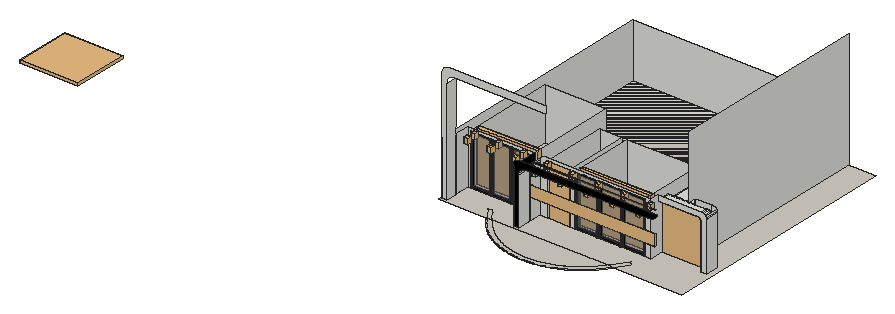
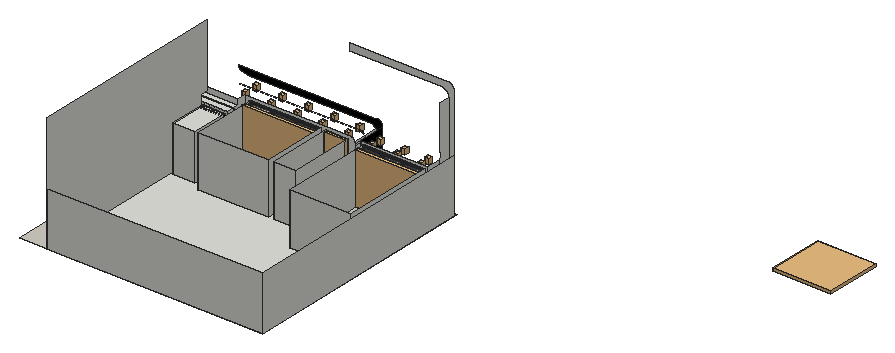
# SketchUp Ruby script. Lengths in inches.
U = 1.inch
M = Sketchup.active_model
def pt(a) = Geom::Point3d.new(a.map { |v| v * U })
def face(e, loops, mat)
  f = e.add_face(loops[0].map { |a| pt(a) })
  loops[1..].each { |l| e.add_face(l.map { |a| pt(a) }).erase! }
  f.material = f.back_material = mat if mat
  f
end
# faces: each face lists its corners as indices into pts; further lists are holes
def faces(e, pts, list, mat = nil) = list.each { |f| face(e, (f[0].is_a?(Array) ? f : [f]).map { |l| l.map { |i| pts[i] } }, mat) }
# xy, xz, yz: faces in a plane at the given z, y or x. An outline is a flat list of corners, or four numbers for a rectangle; further outlines are holes
def ring(l) = l.size == 4 ? [[l[0], l[1]], [l[2], l[1]], [l[2], l[3]], [l[0], l[3]]] : l.each_slice(2).to_a
def flat(e, list, mat, &to3) = list.each { |f| face(e, (f[0].is_a?(Array) ? f : [f]).map { |l| ring(l).map { |u, v| to3.(u, v) } }, mat) }
def xy(e, z, list, mat = nil) = flat(e, list, mat) { |x, y| [x, y, z] }
def xz(e, y, list, mat = nil) = flat(e, list, mat) { |x, z| [x, y, z] }
def yz(e, x, list, mat = nil) = flat(e, list, mat) { |y, z| [x, y, z] }
def lines(e, pts, list) = list.each { |a, b| e.add_line(pt(pts[a]), pt(pts[b])) }
# prism: a flat outline (further loops are holes) pulled along v
def prism(e, loops, v, mat = nil)
  f = face(e, loops, mat); d = Geom::Vector3d.new(v.map { |x| x * U })
  f.pushpull(f.normal.samedirection?(d) ? d.length : -d.length)
end
def box(e, o, s, mat = nil) = prism(e, [[o, [o[0] + s[0], o[1], o[2]], [o[0] + s[0], o[1] + s[1], o[2]], [o[0], o[1] + s[1], o[2]]]], [0, 0, s[2]], mat)
def at(x, y, z, deg = 0) = Geom::Transformation.translation(pt([x, y, z])) * Geom::Transformation.rotation(ORIGIN, Z_AXIS, deg.degrees)
def axes(o, x, y, z) = Geom::Transformation.new([*x, 0, *y, 0, *z, 0, *pt(o).to_a, 1])
def part(name) = M.definitions.add(name)
# library, detail: a bought-in or finely detailed component or shape, given as its bounding box
def library(name, o, s) = part(name).tap { |d| box(d.entities, o, s) }
def detail(e, o, s) = box(e.add_group.entities, o, s)
def put(e, d, t, mat = nil) = e.add_instance(d, t).tap { |i| i.material = mat if mat }
def group(e, t, mat = nil) = e.add_group.tap { |g| g.transformation = t; g.material = mat if mat }.entities
root = M.entities
M.materials.add("Arta-Ceramic-Moonstone-White-24x24-4K").color = [209, 205, 196]
M.materials.add("Glass_Tinted_Gray").color = [0, 0, 0]
M.materials["Glass_Tinted_Gray"].alpha = 0.125
M.materials.add("[0130_Gainsboro]").color = [39, 45, 50]
M.materials.add("[0135_DarkGray]").color = [81, 81, 81]
M.materials.add("[Color M00]").color = [255, 255, 255]
M.materials.add("[Color M09]").color = [0, 0, 0]
M.materials.add("[Mirror 02]").color = [229, 229, 229]
M.materials.add("[Terrazzo Light Blue]").color = [196, 214, 227]
M.materials.add("[Translucent Glass Gray]1").color = [128, 128, 128]
M.materials["[Translucent Glass Gray]1"].alpha = 0.5
c1 = library("CURTAIN",[20.4,9.88,0],[29.77,2.88,102.36])
c2 = library("door by lz",[5.91,-4.92,0],[35.43,6.61,78.74])
c3 = library("Mesh Light\#2",[-0.5,-0.5,-0.1],[1,1,0.2])
c4 = library("Group\#4",[-0.5,-0.5,0],[98.5,2,108])
c5 = part("Glazed door panel")
xy(c5.entities,0,[[0,-0.98,43.07,0],[0,0,43.07,1.4]],"[0130_Gainsboro]")
xy(c5.entities,0.3,[[0.3,-1.43,42.77,-0.98]],"[0130_Gainsboro]")
xy(c5.entities,2.95,[[2.95,-0.63,40.12,0],[2.95,0,40.12,0.64],[2.95,0.64,40.12,1.4]],"[0130_Gainsboro]")
xy(c5.entities,2.95,[[2.95,-1.43,40.12,-0.63]],"[Color M09]")
xy(c5.entities,3.54,[[3.54,0,39.53,0.64]],"[0130_Gainsboro]")
xy(c5.entities,3.54,[[3.54,-0.63,39.53,0]],"[Color M09]")
xy(c5.entities,111.8125,[[3.54,0,39.53,0.64]],"[0130_Gainsboro]")
xy(c5.entities,111.8125,[[3.54,-0.63,39.53,0]],"[Color M09]")
xy(c5.entities,112.4,[[2.95,-0.63,40.12,0],[2.95,0,40.12,0.64],[2.95,0.64,40.12,1.4]],"[0130_Gainsboro]")
xy(c5.entities,112.4,[[2.95,-1.43,40.12,-0.63]],"[Color M09]")
xy(c5.entities,115.05,[[0.3,-1.43,42.77,-0.98]],"[0130_Gainsboro]")
xy(c5.entities,115.35,[[0,-0.98,43.07,0],[0,0,43.07,1.4]],"[0130_Gainsboro]")
xz(c5.entities,-1.43,[[[0.3,0.3,42.77,115.05],[2.95,2.95,40.12,112.4]]],"[Color M09]")
xz(c5.entities,-0.98,[[[0,0,43.07,115.35],[0.3,0.3,42.77,115.05]]],"[Color M00]")
xz(c5.entities,-0.63,[[[2.95,2.95,40.12,112.4],[3.54,3.54,39.53,111.8125]]],"[Color M09]")
xz(c5.entities,0,[[[0,0,43.07,115.35],[2.95,2.95,40.12,112.4]],[[2.95,2.95,40.12,112.4],[3.54,3.54,39.53,111.8125]]],"[0130_Gainsboro]")
xz(c5.entities,0,[[3.54,3.54,39.53,111.8125]],"[Translucent Glass Gray]1")
xz(c5.entities,0.64,[[[2.95,2.95,40.12,112.4],[3.54,3.54,39.53,111.8125]]],"[0130_Gainsboro]")
xz(c5.entities,1.4,[[[0,0,43.07,115.35],[2.95,2.95,40.12,112.4]]],"[0130_Gainsboro]")
yz(c5.entities,0,[[-0.98,0,0,115.35],[0,0,1.4,115.35]],"[0130_Gainsboro]")
yz(c5.entities,0.3,[[-1.43,0.3,-0.98,115.05]],"[Color M00]")
yz(c5.entities,2.95,[[-0.63,2.95,0,112.4],[0,2.95,0.64,112.4],[0.64,2.95,1.4,112.4]],"[0130_Gainsboro]")
yz(c5.entities,2.95,[[-1.43,2.95,-0.63,112.4]],"[Color M09]")
yz(c5.entities,3.54,[[0,3.54,0.64,111.8125]],"[0130_Gainsboro]")
yz(c5.entities,3.54,[[-0.63,3.54,0,111.8125]],"[Color M09]")
yz(c5.entities,39.53,[[0,3.54,0.64,111.8125]],"[0130_Gainsboro]")
yz(c5.entities,39.53,[[-0.63,3.54,0,111.8125]],"[Color M09]")
yz(c5.entities,40.12,[[-0.63,2.95,0,112.4],[0,2.95,0.64,112.4],[0.64,2.95,1.4,112.4]],"[0130_Gainsboro]")
yz(c5.entities,40.12,[[-1.43,2.95,-0.63,112.4]],"[Color M09]")
yz(c5.entities,42.77,[[-1.43,0.3,-0.98,115.05]],"[Color M00]")
yz(c5.entities,43.07,[[-0.98,0,0,115.35],[0,0,1.4,115.35]],"[0130_Gainsboro]")
c6 = part("Sliding glass doors")
put(c6.entities,c5,axes([90.57,1.43,0],[1.05148,0,0],[0,1,0],[0,0,1]),"[Color M09]")
put(c6.entities,c5,axes([0,1.43,0],[1.05148,0,0],[0,1,0],[0,0,1]))
put(c6.entities,c5,axes([45.29,1.43,0],[1.05148,0,0],[0,1,0],[0,0,1]))
c7 = part("PENTEK_RP Fineline 50S_Sliding_DoorCase_E1")
xy(c7.entities,0,[[0,0,1.51,3.66]],"[Color M09]")
xy(c7.entities,99.27,[[0,0,1.51,3.66]],"[Color M09]")
xz(c7.entities,0,[[0,0,1.51,99.27]],"[Color M09]")
xz(c7.entities,3.66,[[0,0,1.51,99.27]],"[0135_DarkGray]")
yz(c7.entities,0,[[0,0,3.66,99.27]],"[Color M09]")
yz(c7.entities,1.51,[[0,0,3.66,99.27]],"[Color M09]")
c8 = part("PENTEK_RP Fineline 50S_SlidingDooe_Case_E2")
xy(c8.entities,0,[[0,0,96.25,3.66]],"[Color M09]")
xy(c8.entities,1.51,[[0,0,96.25,3.66]],"[Color M09]")
xz(c8.entities,0,[[0,0,96.25,1.51]],"[Color M09]")
xz(c8.entities,3.66,[[0,0,96.25,1.51]],"[0135_DarkGray]")
yz(c8.entities,0,[[0,0,3.66,1.51]],"[Color M09]")
yz(c8.entities,96.25,[[0,0,3.66,1.51]],"[Color M09]")
c9 = part("pentek_RP Fineline 50S_SlidingDoor_Case")
put(c9.entities,c7,at(97.76,0,0))
put(c9.entities,c8,at(1.51,0,0))
put(c9.entities,c7,at(0,0,0))
put(c9.entities,c8,at(1.51,0,97.76))
c10 = part("PENTEK_RP Fineline 50S_SlidingDoor_GlazingBead_2")
xy(c10.entities,0,[[0,0,0.56,0.59]],"[0135_DarkGray]")
xy(c10.entities,94.39,[[0,0,0.56,0.59]],"[0135_DarkGray]")
xz(c10.entities,0,[[0,0,0.56,94.39]],"[Color M09]")
xz(c10.entities,0.59,[[0,0,0.56,94.39]],"[0135_DarkGray]")
yz(c10.entities,0,[[0,0,0.59,94.39]],"[0135_DarkGray]")
yz(c10.entities,0.56,[[0,0,0.59,94.39]],"[Color M09]")
c11 = part("PENTEK_RP Fineline 50S_SlidingDoor_Glass")
box(c11.entities,[0,0,0],[46.58,0.16,94.39],"Glass_Tinted_Gray")
c12 = part("PENTEK_RP Fineline 50S_SlidingDoor_GlazingBead")
box(c12.entities,[0,0,0],[45.47,0.59,0.56],"[Color M09]")
c13 = part("PENTEK_RP Fineline 50S_SlidingDoor_Leaf_E1")
xy(c13.entities,0,[[0,0,0.93,1.97],[0.93,1.57,1.49,1.97]],"[0135_DarkGray]")
xy(c13.entities,96.25,[[0,0,0.93,0,0.93,1.57,1.49,1.57,1.49,1.97,0,1.97]],"[0135_DarkGray]")
xz(c13.entities,0,[[0,0,0.93,96.25]],"[Color M09]")
xz(c13.entities,1.57,[[0.93,0,1.49,95.32],[0.93,95.32,1.49,96.25]],"[0135_DarkGray]")
xz(c13.entities,1.97,[[0,0,1.49,96.25]],"[0135_DarkGray]")
yz(c13.entities,0,[[0,0,1.97,96.25]],"[Color M09]")
yz(c13.entities,0.93,[[0,0,1.57,0.93],[0,95.32,1.57,96.25]],"[0135_DarkGray]")
yz(c13.entities,0.93,[[0,0.93,1.57,95.32]],"[Color M09]")
yz(c13.entities,1.49,[[1.57,0,1.97,95.32],[1.57,95.32,1.97,96.25]],"[0135_DarkGray]")
c14 = part("PENTEK_RP Fineline 50S_SlidingDoor_Leaf_E2")
xy(c14.entities,0,[[0,0,0,1.57,0.56,1.57,0.56,1.97,46.02,1.97,46.02,1.57,46.58,1.57,46.58,0]],"[Color M09]")
xy(c14.entities,0.93,[[0,0,46.58,1.57]],"[Color M09]")
xy(c14.entities,1.49,[[0.56,1.57,46.02,1.97]],"[Color M09]")
xz(c14.entities,0,[[0,0,46.58,0.93]],"[Color M09]")
xz(c14.entities,1.57,[[0,0,0.56,0.93],[46.02,0,46.58,0.93]],"[0135_DarkGray]")
xz(c14.entities,1.57,[[0.56,0.93,46.02,1.49]],"[Color M09]")
xz(c14.entities,1.97,[[0.56,0,46.02,1.49]],"[0135_DarkGray]")
yz(c14.entities,0,[[0,0,1.57,0.93]],"[Color M09]")
yz(c14.entities,0.56,[[1.57,0,1.97,0.93]],"[0135_DarkGray]")
yz(c14.entities,0.56,[[1.57,0.93,1.97,1.49]],"[Color M09]")
yz(c14.entities,46.02,[[1.57,0,1.97,0.93]],"[0135_DarkGray]")
yz(c14.entities,46.02,[[1.57,0.93,1.97,1.49]],"[Color M09]")
yz(c14.entities,46.58,[[0,0,1.57,0.93]],"[Color M09]")
c15 = part("PENTEK_RP Fineline S_SlidingDoor_Leaf1")
put(c15.entities,c10,at(0.93,0,0.93))
put(c15.entities,c10,at(46.96,0,0.93))
put(c15.entities,c11,at(1.49,1.42,0.93))
put(c15.entities,c12,at(1.49,0,0.93))
put(c15.entities,c11,at(1.49,0.59,0.93),"[Terrazzo Light Blue]")
put(c15.entities,c13,at(0,0,0))
put(c15.entities,c13,axes([48.44,0,0],[-1,0,0],[0,1,0],[0,0,1]))
put(c15.entities,c14,axes([0.93,0,96.25],[1,0,0],[0,1,0],[0,0,-1]))
put(c15.entities,c14,at(0.93,0,0))
put(c15.entities,c12,at(1.49,0,94.77))
c16 = part("PENTEK_RP Fineline 50S_SlidingDoor_Leaf2")
put(c16.entities,c11,at(1.49,1.42,0.93))
put(c16.entities,c12,at(1.49,0,94.77))
put(c16.entities,c10,at(46.96,0,0.93))
put(c16.entities,c11,at(1.49,0.59,0.93),"[Mirror 02]")
put(c16.entities,c10,at(0.93,0,0.93))
put(c16.entities,c13,at(0,0,0))
put(c16.entities,c13,axes([48.44,0,0],[-1,0,0],[0,1,0],[0,0,1]))
put(c16.entities,c12,at(1.49,0,0.93))
put(c16.entities,c14,axes([0.93,0,96.25],[1,0,0],[0,1,0],[0,0,-1]))
put(c16.entities,c14,at(0.93,0,0))
c17 = part("PENTEK - Slimmest Steel Sliding Door / Window\#2")
put(c17.entities,c9,at(0,-1.88,-0.09),"[Color M09]")
put(c17.entities,c15,at(1.51,-2.27,1.42))
put(c17.entities,c16,at(49.32,-0.3,1.42))
c18 = library("Curtains",[0,0,0],[121.73,8.19,117.22])
c19 = library("Group\#166",[0,0,0],[129,124.5,6])
c20 = library("IES Light",[-4.45,-4.45,-12],[8.9,8.9,12])
xy(root,30,[[777.4375,202.125,777.4375,734.875,1257.4375,734.875,1257.4375,307.9375,1251.4375,307.9375,1251.4375,391.375,1202.71,391.375,1202.71,307.9375,1196.71,307.9375,1196.71,260.875,1183.9375,260.875,1183.9375,406.0625,1027.75,406.0625,1027.75,260.875,1015.75,260.875,1015.75,406.0625,967.75,406.0625,967.75,260.875,949.4375,260.875,949.4375,202.125,937.4375,202.125,937.4375,260.875,931.4375,260.875,931.4375,467.3125,795.4375,467.3125,795.4375,260.875,789.4375,260.875,789.4375,202.125],[1294.21,278.875,1306.21,307.9375]])
xy(root,30,[[1024.28,117.49,1027.49,117.52,1030.7,117.61,1033.91,117.77,1037.12,117.98,1040.32,118.26,1043.51,118.6,1046.7,119,1049.88,119.46,1053.05,119.98,1056.21,120.5625,1059.36,121.2,1062.49,121.91,1065.61,122.67,1068.72,123.49,1071.81,124.375,1074.875,125.32,1077.93,126.32,1080.96,127.375,1083.97,128.49,1086.97,129.67,1089.93,130.9,1092.875,132.1875,1095.79,133.53,1098.68,134.93,1101.55,136.38,1104.38,137.89,1107.19,139.46,1109.97,141.08,1112.71,142.75,1115.42,144.47,1118.1,146.24,1120.74,148.07,1123.35,149.94,1125.92,151.87,1128.46,153.84,1130.95,155.87,1133.41,157.9375,1135.82,160.05,1138.2,162.22,1140.53,164.43,1142.82,166.68,1145.07,168.97,1147.27,171.3125,1149.43,173.69,1151.54,176.12,1153.6,178.58,1155.62,181.08,1157.59,183.62,1159.51,186.19,1165.71,194.86,1165.69,194.875,1164.72,194.875,1158.85,186.67,1156.94,184.11,1154.98,181.58,1152.97,179.09,1150.92,176.64,1148.82,174.23,1146.67,171.87,1144.48,169.54,1142.25,167.25,1139.97,165.01,1137.64,162.8125,1135.28,160.66,1132.875,158.55,1130.43,156.49,1127.95,154.48,1125.43,152.52,1122.87,150.6,1120.27,148.73,1117.64,146.92,1114.98,145.15,1112.28,143.4375,1109.55,141.77,1106.79,140.16,1103.99,138.61,1101.17,137.11,1098.32,135.66,1095.45,134.27,1092.54,132.93,1089.61,131.65,1086.66,130.42,1083.68,129.25,1080.6875,128.14,1077.67,127.09,1074.63,126.09,1071.57,125.16,1068.5,124.28,1065.41,123.46,1062.31,122.7,1059.1875,122,1056.05,121.36,1052.91,120.78,1049.76,120.26,1046.59,119.8,1043.42,119.41,1040.24,119.07,1037.06,118.79,1033.87,118.58,1030.67,118.43,1027.48,118.33,1024.28,118.3,1021.08,118.33,1017.89,118.43,1014.7,118.58,1011.51,118.79,1008.32,119.07,1005.14,119.41,1001.97,119.8,998.81,120.26,995.65,120.78,992.51,121.36,989.375,122,986.26,122.7,983.15,123.46,980.0625,124.28,976.99,125.16,973.93,126.09,970.89,127.09,967.875,128.14,964.875,129.25,961.9,130.42,958.95,131.65,956.02,132.93,953.12,134.27,950.24,135.66,947.39,137.11,944.57,138.61,941.77,140.16,939.01,141.77,936.28,143.4375,933.58,145.15,930.92,146.92,928.29,148.73,925.69,150.6,923.13,152.52,920.61,154.48,918.13,156.49,915.68,158.55,913.28,160.66,910.92,162.8125,908.59,165.01,906.32,167.25,904.08,169.54,901.89,171.87,899.74,174.23,897.64,176.64,895.59,179.09,893.58,181.58,891.62,184.11,889.71,186.67,883.84,194.875,882.84,194.875,889.06,186.19,890.97,183.62,892.94,181.08,894.96,178.58,897.02,176.12,899.13,173.69,901.29,171.3125,903.49,168.97,905.74,166.68,908.03,164.43,910.36,162.22,912.74,160.05,915.15,157.9375,917.61,155.87,920.11,153.84,922.64,151.87,925.21,149.94,927.82,148.07,930.46,146.24,933.14,144.47,935.85,142.75,938.6,141.08,941.37,139.46,944.18,137.89,947.01,136.38,949.88,134.93,952.77,133.53,955.6875,132.1875,958.63,130.9,961.6,129.67,964.59,128.49,967.6,127.375,970.63,126.32,973.68,125.32,976.76,124.375,979.85,123.49,982.95,122.67,986.07,121.91,989.21,121.2,992.35,120.5625,995.51,119.98,998.68,119.46,1001.86,119,1005.05,118.6,1008.24,118.26,1011.44,117.98,1014.65,117.77,1017.86,117.61,1021.07,117.52],[1024.28,118.3,1027.48,118.33,1030.67,118.43,1033.87,118.58,1037.06,118.79,1040.24,119.07,1043.42,119.41,1046.59,119.8,1049.76,120.26,1052.91,120.78,1056.05,121.36,1059.1875,122,1062.31,122.7,1065.41,123.46,1068.5,124.28,1071.57,125.16,1074.63,126.09,1077.67,127.09,1080.6875,128.14,1083.68,129.25,1086.66,130.42,1089.61,131.65,1092.54,132.93,1095.45,134.27,1098.32,135.66,1101.17,137.11,1103.99,138.61,1106.79,140.16,1109.55,141.77,1112.28,143.4375,1114.98,145.15,1117.64,146.92,1120.27,148.73,1122.87,150.6,1125.43,152.52,1127.95,154.48,1130.43,156.49,1132.875,158.55,1135.28,160.66,1137.64,162.8125,1139.97,165.01,1142.25,167.25,1144.48,169.54,1146.67,171.87,1148.82,174.23,1150.92,176.64,1152.97,179.09,1154.98,181.58,1156.94,184.11,1158.85,186.67,1164.72,194.875,1152.72,194.875,1150.98,192.41,1149.2,189.97,1147.37,187.57,1145.49,185.21,1143.57,182.88,1141.61,180.59,1139.59,178.34,1137.54,176.125,1135.45,173.95,1133.31,171.82,1131.13,169.73,1128.91,167.6875,1126.65,165.68,1124.36,163.72,1122.02,161.81,1119.65,159.94,1117.25,158.12,1114.81,156.34,1112.33,154.61,1109.83,152.93,1107.29,151.3,1104.72,149.72,1102.12,148.19,1099.49,146.71,1096.83,145.28,1094.14,143.9,1091.43,142.57,1088.69,141.3,1085.93,140.08,1083.15,138.91,1080.34,137.8,1077.52,136.74,1074.67,135.74,1071.81,134.79,1068.92,133.9,1066.02,133.07,1063.11,132.29,1060.18,131.5625,1057.23,130.9,1054.28,130.29,1051.31,129.74,1048.33,129.24,1045.34,128.81,1042.35,128.43,1039.35,128.11,1036.34,127.84,1033.33,127.64,1030.32,127.49,1027.3,127.41,1024.28,127.375,1021.26,127.41,1018.25,127.49,1015.23,127.64,1012.22,127.84,1009.21,128.11,1006.21,128.43,1003.22,128.81,1000.23,129.24,997.25,129.74,994.29,130.29,991.33,130.9,988.39,131.5625,985.46,132.29,982.54,133.07,979.64,133.9,976.76,134.79,973.89,135.74,971.04,136.74,968.22,137.8,965.41,138.91,962.63,140.08,959.87,141.3,957.13,142.57,954.42,143.9,951.73,145.28,949.08,146.71,946.45,148.19,943.85,149.72,941.27,151.3,938.74,152.93,936.23,154.61,933.75,156.34,931.3125,158.12,928.91,159.94,926.54,161.81,924.2,163.72,921.91,165.68,919.65,167.6875,917.43,169.73,915.25,171.82,913.12,173.95,911.02,176.125,908.97,178.34,906.96,180.59,904.99,182.88,903.07,185.21,901.19,187.57,899.36,189.97,897.58,192.41,895.84,194.875,883.84,194.875,889.71,186.67,891.62,184.11,893.58,181.58,895.59,179.09,897.64,176.64,899.74,174.23,901.89,171.87,904.08,169.54,906.32,167.25,908.59,165.01,910.92,162.8125,913.28,160.66,915.68,158.55,918.13,156.49,920.61,154.48,923.13,152.52,925.69,150.6,928.29,148.73,930.92,146.92,933.58,145.15,936.28,143.4375,939.01,141.77,941.77,140.16,944.57,138.61,947.39,137.11,950.24,135.66,953.12,134.27,956.02,132.93,958.95,131.65,961.9,130.42,964.875,129.25,967.875,128.14,970.89,127.09,973.93,126.09,976.99,125.16,980.0625,124.28,983.15,123.46,986.26,122.7,989.375,122,992.51,121.36,995.65,120.78,998.81,120.26,1001.97,119.8,1005.14,119.41,1008.32,119.07,1011.51,118.79,1014.7,118.58,1017.89,118.43,1021.08,118.33],[1024.28,127.375,1027.3,127.41,1030.32,127.49,1033.33,127.64,1036.34,127.84,1039.35,128.11,1042.35,128.43,1045.34,128.81,1048.33,129.24,1051.31,129.74,1054.28,130.29,1057.23,130.9,1060.18,131.5625,1063.11,132.29,1066.02,133.07,1068.92,133.9,1071.81,134.79,1074.67,135.74,1077.52,136.74,1080.34,137.8,1083.15,138.91,1085.93,140.08,1088.69,141.3,1091.43,142.57,1094.14,143.9,1096.83,145.28,1099.49,146.71,1102.12,148.19,1104.72,149.72,1107.29,151.3,1109.83,152.93,1112.33,154.61,1114.81,156.34,1117.25,158.12,1119.65,159.94,1122.02,161.81,1124.36,163.72,1126.65,165.68,1128.91,167.6875,1131.13,169.73,1133.31,171.82,1135.45,173.95,1137.54,176.125,1139.59,178.34,1141.61,180.59,1143.57,182.88,1145.49,185.21,1147.37,187.57,1149.2,189.97,1150.98,192.41,1152.72,194.875,1150.97,192.43,1149.17,190.01,1147.33,187.64,1145.4375,185.29,1143.5,182.99,1141.52,180.72,1139.5,178.49,1137.44,176.3,1135.34,174.15,1133.19,172.04,1131,169.97,1128.78,167.94,1126.52,165.96,1124.21,164.02,1121.875,162.12,1119.5,160.27,1117.09,158.47,1114.65,156.71,1112.17,155,1109.67,153.34,1107.125,151.72,1104.55,150.16,1101.95,148.64,1099.33,147.18,1096.67,145.76,1093.99,144.4,1091.28,143.09,1088.54,141.83,1085.79,140.625,1083.01,139.47,1080.21,138.37,1077.38,137.32,1074.54,136.33,1071.68,135.4,1068.8,134.51,1065.91,133.6875,1063,132.92,1060.08,132.2,1057.14,131.54,1054.19,130.94,1051.23,130.4,1048.26,129.91,1045.28,129.48,1042.3,129.1,1039.31,128.78,1036.31,128.52,1033.3,128.32,1030.3,128.18,1027.29,128.09,1024.28,128.0625,1021.27,128.09,1018.26,128.18,1015.26,128.32,1012.25,128.52,1009.26,128.78,1006.26,129.1,1003.28,129.48,1000.3,129.91,997.33,130.4,994.37,130.94,991.42,131.54,988.48,132.2,985.56,132.92,982.65,133.6875,979.76,134.51,976.88,135.4,974.02,136.33,971.18,137.32,968.36,138.37,965.56,139.47,962.78,140.625,960.02,141.83,957.28,143.09,954.58,144.4,951.89,145.76,949.24,147.18,946.61,148.64,944.01,150.16,941.4375,151.72,938.9,153.34,936.39,155,933.91,156.71,931.47,158.47,929.06,160.27,926.69,162.12,924.35,164.02,922.05,165.96,919.78,167.94,917.56,169.97,915.37,172.04,913.23,174.15,911.12,176.3,909.06,178.49,907.04,180.72,905.06,182.99,903.125,185.29,901.24,187.64,899.39,190.01,897.59,192.43,895.84,194.875,897.58,192.41,899.36,189.97,901.19,187.57,903.07,185.21,904.99,182.88,906.96,180.59,908.97,178.34,911.02,176.125,913.12,173.95,915.25,171.82,917.43,169.73,919.65,167.6875,921.91,165.68,924.2,163.72,926.54,161.81,928.91,159.94,931.3125,158.12,933.75,156.34,936.23,154.61,938.74,152.93,941.27,151.3,943.85,149.72,946.45,148.19,949.08,146.71,951.73,145.28,954.42,143.9,957.13,142.57,959.87,141.3,962.63,140.08,965.41,138.91,968.22,137.8,971.04,136.74,973.89,135.74,976.76,134.79,979.64,133.9,982.54,133.07,985.46,132.29,988.39,131.5625,991.33,130.9,994.29,130.29,997.25,129.74,1000.23,129.24,1003.22,128.81,1006.21,128.43,1009.21,128.11,1012.22,127.84,1015.23,127.64,1018.25,127.49,1021.26,127.41],[1024.28,128.0625,1027.29,128.09,1030.3,128.18,1033.3,128.32,1036.31,128.52,1039.31,128.78,1042.3,129.1,1045.28,129.48,1048.26,129.91,1051.23,130.4,1054.19,130.94,1057.14,131.54,1060.08,132.2,1063,132.92,1065.91,133.6875,1068.8,134.51,1071.68,135.4,1074.54,136.33,1077.38,137.32,1080.21,138.37,1083.01,139.47,1085.79,140.625,1088.54,141.83,1091.28,143.09,1093.99,144.4,1096.67,145.76,1099.33,147.18,1101.95,148.64,1104.55,150.16,1107.125,151.72,1109.67,153.34,1112.17,155,1114.65,156.71,1117.09,158.47,1119.5,160.27,1121.875,162.12,1124.21,164.02,1126.52,165.96,1128.78,167.94,1131,169.97,1133.19,172.04,1135.34,174.15,1137.44,176.3,1139.5,178.49,1141.52,180.72,1143.5,182.99,1145.4375,185.29,1147.33,187.64,1149.17,190.01,1150.97,192.43,1152.72,194.875,895.84,194.875,897.59,192.43,899.39,190.01,901.24,187.64,903.125,185.29,905.06,182.99,907.04,180.72,909.06,178.49,911.12,176.3,913.23,174.15,915.37,172.04,917.56,169.97,919.78,167.94,922.05,165.96,924.35,164.02,926.69,162.12,929.06,160.27,931.47,158.47,933.91,156.71,936.39,155,938.9,153.34,941.4375,151.72,944.01,150.16,946.61,148.64,949.24,147.18,951.89,145.76,954.58,144.4,957.28,143.09,960.02,141.83,962.78,140.625,965.56,139.47,968.36,138.37,971.18,137.32,974.02,136.33,976.88,135.4,979.76,134.51,982.65,133.6875,985.56,132.92,988.48,132.2,991.42,131.54,994.37,130.94,997.33,130.4,1000.3,129.91,1003.28,129.48,1006.26,129.1,1009.26,128.78,1012.25,128.52,1015.26,128.32,1018.26,128.18,1021.27,128.09],[777.4375,194.875,882.84,194.875,882.57,195.26,883.23,195.73,865.83,220.05,873.77,225.73,895.84,194.875,1152.72,194.875,1177.16,229.03,1185.09,223.35,1165.05,195.33,1165.69,194.875,1318.21,194.875,1318.21,734.875,777.4375,734.875],
  [883.84,194.875,895.84,194.875,873.77,225.73,865.83,220.05,883.23,195.73],[882.84,194.875,883.84,194.875,883.23,195.73,882.57,195.26],[1152.72,194.875,1164.72,194.875,1165.05,195.33,1185.09,223.35,1177.16,229.03],[1164.72,194.875,1165.69,194.875,1165.05,195.33]],"Arta-Ceramic-Moonstone-White-24x24-4K")
xy(root,132,[[1202.71,307.9375,1251.4375,391.375]])
xy(root,138,[[1196.71,278.875,1282.21,291.4375],[1196.71,292.4375,1282.21,307.9375]])
xz(root,202.125,[[777.4375,30,789.4375,30,789.4375,261.71,789.92,266.99,791.36,271.3125,793.76,274.68,797.125,277.08,801.45,278.52,806.73,279,1009.83,279,1009.83,294,794.73,294,789.45,293.52,785.125,292.08,781.76,289.68,779.36,286.3125,777.92,281.99,777.4375,276.71]])
xz(root,202.125,[[937.4375,30,949.4375,30,949.4375,135.83,949.83,140.16,951.01,143.7,952.98,146.46,955.74,148.43,959.28,149.61,963.61,150,1228.2,150,1237.13,150.39,1244.44,151.54,1250.13,153.47,1254.1875,156.17,1256.625,159.64,1257.4375,163.875,951.61,163.875,947.28,163.48,943.74,162.3,940.98,160.33,939.01,157.58,937.83,154.03,937.4375,149.7]],"[Color M09]")
xz(root,260.875,[[789.4375,30,795.4375,30,795.4375,144,931.4375,144,931.4375,30,937.4375,30,937.4375,150,789.4375,150],[949.4375,30,967.75,30,967.75,143.7,1015.75,143.7,1015.75,30,1027.75,30,1027.75,143.7,1183.9375,143.7,1183.9375,30,1196.71,30,1196.71,150,963.61,150,959.28,149.61,955.74,148.43,952.98,146.46,951.01,143.7,949.83,140.16,949.4375,135.83]])
xz(root,278.875,[[1294.21,30,1306.21,30,1306.21,138,1305.88,141.67,1304.88,144.67,1303.21,147,1300.88,148.67,1297.88,149.67,1294.21,150,1196.71,150,1196.71,138,1282.21,138,1285.88,137.67,1288.88,136.67,1291.21,135,1292.88,132.67,1293.88,129.67,1294.21,126]])
xz(root,307.9375,[[1196.71,30,1202.71,30,1202.71,132,1251.4375,132,1251.4375,30,1257.4375,30,1257.4375,138,1196.71,138],[1294.21,30,1294.21,150,1297.88,149.67,1300.88,148.67,1303.21,147,1304.88,144.67,1305.88,141.67,1306.21,138,1306.21,30],[1294.21,126,1293.88,129.67,1292.88,132.67,1291.21,135,1288.88,136.67,1285.88,137.67,1282.21,138,1294.21,138],[1257.4375,138,1294.21,150]])
xz(root,391.375,[[1202.71,30,1251.4375,132]])
xz(root,406.0625,[[967.75,30,1015.75,143.7],[1027.75,30,1183.9375,143.7]])
xz(root,467.3125,[[795.4375,30,931.4375,144]])
xz(root,734.875,[[777.4375,30,1257.4375,150]])
yz(root,777.4375,[[202.125,30,734.875,150]])
yz(root,789.4375,[[202.125,30,226.5,30,226.5,150,224.875,150,224.875,163.875,226.5,163.875,226.5,261.71,202.125,261.71],[226.5,30,227.5,150],[227.5,30,260.875,150]])
yz(root,795.4375,[[260.875,30,467.3125,144]])
yz(root,931.4375,[[260.875,30,467.3125,144]])
yz(root,937.4375,[[202.125,30,202.125,149.7,224.875,150,260.875,150,260.875,30]],"[Color M09]")
yz(root,949.4375,[[202.125,30,233.0625,135.83],[234.0625,30,260.875,135.83]])
yz(root,967.75,[[260.875,30,406.0625,143.7]])
yz(root,1015.75,[[260.875,30,406.0625,143.7]])
yz(root,1027.75,[[260.875,30,406.0625,143.7]])
yz(root,1183.9375,[[260.875,30,406.0625,143.7]])
yz(root,1196.71,[[260.875,30,307.9375,30,307.9375,138,278.875,138,278.875,150,260.875,150]])
yz(root,1202.71,[[307.9375,30,391.375,132]])
yz(root,1251.4375,[[307.9375,30,391.375,132]])
yz(root,1257.4375,[[307.9375,30,734.875,30,734.875,291,290.7,291,290.7,150,307.9375,150]])
yz(root,1294.21,[[278.875,30,291.4375,126],[292.4375,30,307.9375,126]])
yz(root,1306.21,[[278.875,30,307.9375,138]])
p = [[1293.88,278.875,129.67],[1293.88,291.4375,129.67],[1294.21,291.4375,126],[1294.21,278.875,126],[1294.21,307.9375,126],[1294.21,292.4375,126],
  [1293.88,292.4375,129.67],[1293.88,307.9375,129.67],[1292.88,278.875,132.67],[1292.88,291.4375,132.67],[1292.88,292.4375,132.67],[1292.88,307.9375,132.67],
  [1291.21,278.875,135],[1291.21,291.4375,135],[1291.21,292.4375,135],[1291.21,307.9375,135],[1288.88,278.875,136.67],[1288.88,291.4375,136.67],
  [1288.88,292.4375,136.67],[1288.88,307.9375,136.67],[949.4375,202.125,135.83],[949.4375,233.0625,135.83],[949.83,233.0625,140.16],[949.83,202.125,140.16],
  [949.83,260.875,140.16],[949.83,234.0625,140.16],[949.4375,234.0625,135.83],[949.4375,260.875,135.83],[1285.88,278.875,137.67],[1285.88,291.4375,137.67],
  [1285.88,292.4375,137.67],[1285.88,307.9375,137.67],[1282.21,278.875,138],[1282.21,291.4375,138],[1282.21,292.4375,138],[1282.21,307.9375,138],
  [1306.21,278.875,138],[1306.21,307.9375,138],[1305.88,307.9375,141.67],[1305.88,278.875,141.67],[951.01,233.0625,143.7],[951.01,202.125,143.7],
  [951.01,260.875,143.7],[951.01,234.0625,143.7],[1304.88,307.9375,144.67],[1304.88,278.875,144.67]]
faces(root,p,[[0,1,2,3],[4,5,6,7],[8,9,1,0],[7,6,10,11],[12,13,9,8],[11,10,14,15],[16,17,13,12],[15,14,18,19],
  [20,21,22,23],[24,25,26,27],[28,29,17,16],[19,18,30,31],[32,33,29,28],[31,30,34,35],[36,37,38,39],[23,22,40,41],
  [42,43,25,24],[39,38,44,45]])
put(root,c1,axes([1169.33,305.74,29.64],[1.63653,0,0],[0,1,0],[0,0,1]))
put(root,c2,axes([959.74,266.36,30],[1.35467,0,0],[0,1,0],[0,0,1.44399]))
g1 = group(root,at(949.4375,233.0625,30),"[Color M09]")
xy(g1,120,[[14.17,0,278.56,1]])
yz(g1,0,[[0,0,1,105.83]])
p = [[0.39,1,110.16],[0.39,0,110.16],[0,0,105.83],[0,1,105.83],[1.57,1,113.7],[1.57,0,113.7],
  [3.54,1,116.46],[3.54,0,116.46],[6.3,1,118.43],[6.3,0,118.43],[9.84,1,119.61],[9.84,0,119.61],
  [14.17,1,120],[14.17,0,120]]
faces(g1,p,[[0,1,2,3],[4,5,1,0],[6,7,5,4],[8,9,7,6],[10,11,9,8],[12,13,11,10]])
put(g1,c3,axes([139.28,0.5,60],[279.55874,0,0],[0,2,0],[0,0,121]))
put(root,c4,at(1196.71,291.4375,30))
put(root,c6,axes([796.3125,260.875,30],[0.99458,0,0],[0,1.48574,0],[0,0,0.98826]))
put(root,c6,axes([1028.625,260.875,30],[1.14317,0,0],[0,1.48574,0],[0,0,0.98826]))
put(root,c17,axes([1202.71,310.21,30.09],[0.49081,0,0],[0,1,0],[0,0,1.02748]))
put(root,c18,axes([796.76,276.625,31.73],[1.10639,0,0],[0,1,0],[0,0,0.96]))
put(root,c18,axes([1027.75,275.25,31.73],[1.2831,0,0],[0,1,0],[0,0,0.96]))
put(root,c19,at(0,0,114))
put(root,c20,at(975.9,247.32,149.99))
put(root,c20,at(975.9,216.14,149.99))
put(root,c20,at(1033.46,247.32,149.99))
put(root,c20,at(1033.46,216.14,149.99))
put(root,c20,at(1091.03,247.32,149.99))
put(root,c20,at(1091.03,216.14,149.99))
put(root,c20,at(1148.59,247.32,149.99))
put(root,c20,at(1148.59,216.14,149.99))
put(root,c20,at(1206.15,247.32,149.99))
put(root,c20,at(1206.15,216.14,149.99))
put(root,c20,at(810.48,252.66,150))
put(root,c20,at(810.48,231.66,150))
put(root,c20,at(863.29,231.66,150))
put(root,c20,at(863.29,252.66,150))
put(root,c20,at(918.6,231.66,150))
put(root,c20,at(918.6,252.66,150))
